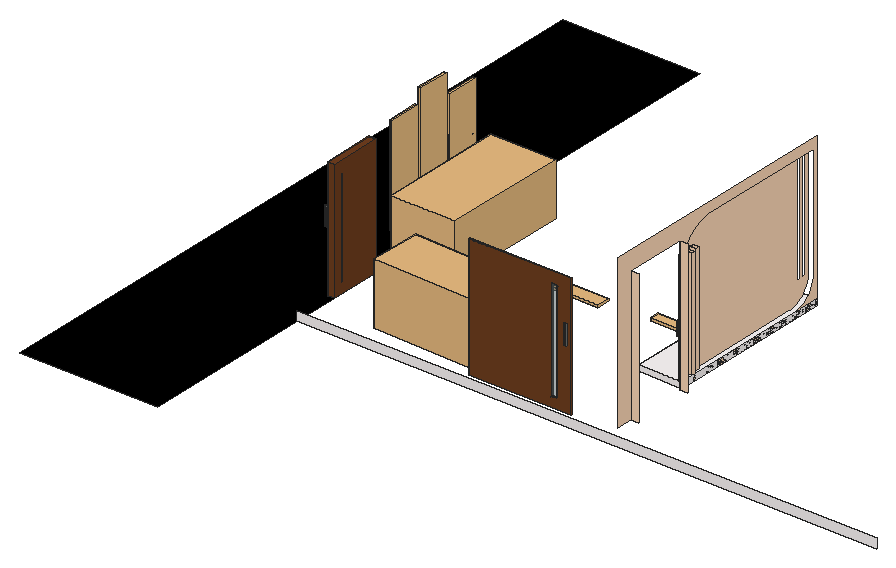
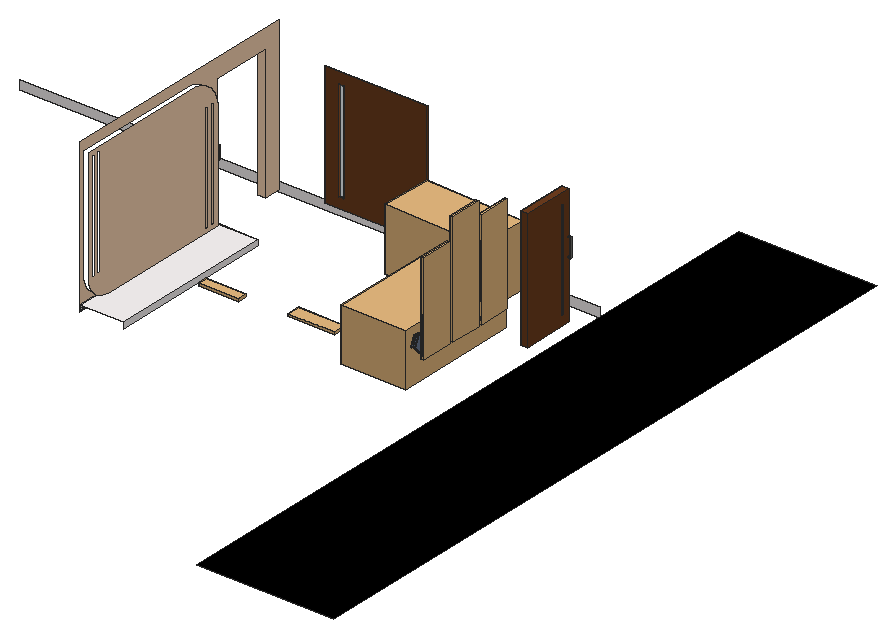
# SketchUp Ruby script. Lengths in inches.
U = 1.inch
M = Sketchup.active_model
def pt(a) = Geom::Point3d.new(a.map { |v| v * U })
def face(e, loops, mat)
  f = e.add_face(loops[0].map { |a| pt(a) })
  loops[1..].each { |l| e.add_face(l.map { |a| pt(a) }).erase! }
  f.material = f.back_material = mat if mat
  f
end
# faces: each face lists its corners as indices into pts; further lists are holes
def faces(e, pts, list, mat = nil) = list.each { |f| face(e, (f[0].is_a?(Array) ? f : [f]).map { |l| l.map { |i| pts[i] } }, mat) }
# xy, xz, yz: faces in a plane at the given z, y or x. An outline is a flat list of corners, or four numbers for a rectangle; further outlines are holes
def ring(l) = l.size == 4 ? [[l[0], l[1]], [l[2], l[1]], [l[2], l[3]], [l[0], l[3]]] : l.each_slice(2).to_a
def flat(e, list, mat, &to3) = list.each { |f| face(e, (f[0].is_a?(Array) ? f : [f]).map { |l| ring(l).map { |u, v| to3.(u, v) } }, mat) }
def xy(e, z, list, mat = nil) = flat(e, list, mat) { |x, y| [x, y, z] }
def xz(e, y, list, mat = nil) = flat(e, list, mat) { |x, z| [x, y, z] }
def yz(e, x, list, mat = nil) = flat(e, list, mat) { |y, z| [x, y, z] }
def lines(e, pts, list) = list.each { |a, b| e.add_line(pt(pts[a]), pt(pts[b])) }
# prism: a flat outline (further loops are holes) pulled along v
def prism(e, loops, v, mat = nil)
  f = face(e, loops, mat); d = Geom::Vector3d.new(v.map { |x| x * U })
  f.pushpull(f.normal.samedirection?(d) ? d.length : -d.length)
end
def box(e, o, s, mat = nil) = prism(e, [[o, [o[0] + s[0], o[1], o[2]], [o[0] + s[0], o[1] + s[1], o[2]], [o[0], o[1] + s[1], o[2]]]], [0, 0, s[2]], mat)
def at(x, y, z, deg = 0) = Geom::Transformation.translation(pt([x, y, z])) * Geom::Transformation.rotation(ORIGIN, Z_AXIS, deg.degrees)
def axes(o, x, y, z) = Geom::Transformation.new([*x, 0, *y, 0, *z, 0, *pt(o).to_a, 1])
def part(name) = M.definitions.add(name)
# library, detail: a bought-in or finely detailed component or shape, given as its bounding box
def library(name, o, s) = part(name).tap { |d| box(d.entities, o, s) }
def detail(e, o, s) = box(e.add_group.entities, o, s)
def put(e, d, t, mat = nil) = e.add_instance(d, t).tap { |i| i.material = mat if mat }
def group(e, t, mat = nil) = e.add_group.tap { |g| g.transformation = t; g.material = mat if mat }.entities
root = M.entities
M.materials.add("3D66_SU_1584934530570_001").color = [198, 166, 120]
M.materials.add("3D66_SU_1584934530605_002").color = [112, 126, 151]
M.materials.add("Material \#1").color = [140, 140, 140]
M.materials.add("[0006_Pink]").color = [255, 192, 203]
M.materials.add("[0010_Snow]").color = [255, 250, 250]
M.materials.add("[0027_PeachPuff]").color = [255, 218, 185]
M.materials.add("[0093_AliceBlue]").color = [240, 248, 255]
M.materials.add("[0137_Black]").color = [0, 0, 0]
M.materials.add("[Metal_Seamed]").color = [118, 119, 115]
M.materials.add("[Translucent_Glass_Safety]").color = [93, 108, 112]
M.materials["[Translucent_Glass_Safety]"].alpha = 0.5
M.materials.add("[Wood_Cherry_Original]").color = [112, 63, 31]
M.materials.add("[Wood_Cherry_Original]1").color = [152, 86, 42]
c1 = part("\#51")
xy(c1.entities,-100.5,[[4942.73,3813.38,5299.1,3883.7]],"3D66_SU_1584934530570_001")
xy(c1.entities,-87.5,[[4944.6875,3815.34,5297.14,3881.74]],"3D66_SU_1584934530570_001")
xz(c1.entities,3813.38,[[4942.73,-100.5,5299.1,-90.5]],"3D66_SU_1584934530570_001")
xz(c1.entities,3883.7,[[4942.73,-100.5,5299.1,-90.5]],"3D66_SU_1584934530570_001")
yz(c1.entities,4942.73,[[3813.38,-100.5,3883.7,-90.5]],"3D66_SU_1584934530570_001")
yz(c1.entities,5299.1,[[3813.38,-100.5,3883.7,-90.5]],"3D66_SU_1584934530570_001")
p = [[4942.73,3883.7,-90.5],[4942.73,3813.38,-90.5],[4944.6875,3815.34,-87.5],[4944.6875,3881.74,-87.5],[5299.1,3813.38,-90.5],[5297.14,3815.34,-87.5],
  [5299.1,3883.7,-90.5],[5297.14,3881.74,-87.5]]
faces(c1.entities,p,[[0,1,2,3],[1,4,5,2],[4,6,7,5],[6,0,3,7]],"3D66_SU_1584934530570_001")
c2 = part("\#48")
xy(c2.entities,-100.5,[[5355.9,3811.42,5712.27,3881.74]],"3D66_SU_1584934530570_001")
xy(c2.entities,-87.5,[[5357.86,3813.38,5710.31,3879.78]],"3D66_SU_1584934530570_001")
xz(c2.entities,3811.42,[[5355.9,-100.5,5712.27,-90.5]],"3D66_SU_1584934530570_001")
xz(c2.entities,3881.74,[[5355.9,-100.5,5712.27,-90.5]],"3D66_SU_1584934530570_001")
yz(c2.entities,5355.9,[[3811.42,-100.5,3881.74,-90.5]],"3D66_SU_1584934530570_001")
yz(c2.entities,5712.27,[[3811.42,-100.5,3881.74,-90.5]],"3D66_SU_1584934530570_001")
p = [[5355.9,3881.74,-90.5],[5355.9,3811.42,-90.5],[5357.86,3813.38,-87.5],[5357.86,3879.78,-87.5],[5712.27,3811.42,-90.5],[5710.31,3813.38,-87.5],
  [5712.27,3881.74,-90.5],[5710.31,3879.78,-87.5]]
faces(c2.entities,p,[[0,1,2,3],[1,4,5,2],[4,6,7,5],[6,0,3,7]],"3D66_SU_1584934530570_001")
c3 = part("\#50")
xy(c3.entities,-100.5,[[4526.8,3811.42,4883.17,3881.74]],"3D66_SU_1584934530570_001")
xy(c3.entities,-87.5,[[4528.76,3813.38,4881.21,3879.78]],"3D66_SU_1584934530570_001")
xz(c3.entities,3811.42,[[4526.8,-100.5,4883.17,-90.5]],"3D66_SU_1584934530570_001")
xz(c3.entities,3881.74,[[4526.8,-100.5,4883.17,-90.5]],"3D66_SU_1584934530570_001")
yz(c3.entities,4526.8,[[3811.42,-100.5,3881.74,-90.5]],"3D66_SU_1584934530570_001")
yz(c3.entities,4883.17,[[3811.42,-100.5,3881.74,-90.5]],"3D66_SU_1584934530570_001")
p = [[4526.8,3881.74,-90.5],[4526.8,3811.42,-90.5],[4528.76,3813.38,-87.5],[4528.76,3879.78,-87.5],[4883.17,3811.42,-90.5],[4881.21,3813.38,-87.5],
  [4883.17,3881.74,-90.5],[4881.21,3879.78,-87.5]]
faces(c3.entities,p,[[0,1,2,3],[1,4,5,2],[4,6,7,5],[6,0,3,7]],"3D66_SU_1584934530570_001")
c4 = library("\#53",[4936.19,3775.67,-115.5],[369.44,1553.17,40])
c5 = part("\#54")
xy(c5.entities,-100.5,[[4523.53,3883.7,4523.53,4334.05,4764.99,3927.74],[4523.53,3883.7,4764.99,3927.74,4784.14,3902.18],[4523.53,3883.7,4784.14,3902.18,4810.21,3883.7],[4810.21,3883.7,4784.14,3902.18,4796.42,3891.95],[4784.14,3902.18,4764.99,3927.74,4773.59,3914.1875],
  [4764.99,3927.74,4523.53,4334.05,4758.58,3942.61],[4758.58,3942.61,4523.53,4334.05,4753.18,3975.46],[4758.58,3942.61,4753.18,3975.46,4754.5625,3958.6],[4753.18,3975.46,4523.53,4334.05,4763.59,4020.47],[4753.18,3975.46,4763.59,4020.47,4755.88,3998.93],
  [4763.59,4020.47,4523.53,4334.05,4791.55,4055.35],[4763.59,4020.47,4791.55,4055.35,4775.6875,4039.49],[4791.55,4055.35,4523.53,4334.05,4810.57,4067.45],[4810.57,4067.45,4523.53,4334.05,4576.49,4391.14],[4810.57,4067.45,4576.49,4391.14,4590.02,4403.74],
  [4810.57,4067.45,4590.02,4403.74,4602.85,4414.71],[4810.57,4067.45,4602.85,4414.71,4615.42,4424.5],[4810.57,4067.45,4615.42,4424.5,4832.11,4075.16],[4886.4375,4072.72,4877.97,4075.17,4886.4375,4525.64],[4886.4375,4072.72,4882.24,4074.03,4877.97,4075.17],
  [4832.11,4075.16,4615.42,4424.5,4621.74,4429.1],[4832.11,4075.16,4621.74,4429.1,4751.37,4455.56],[4832.11,4075.16,4751.37,4455.56,4757.04,4455.48],[4832.11,4075.16,4757.04,4455.48,4855.58,4077.86],[4877.97,4075.17,4869.21,4076.87,4886.4375,4525.64],
  [4877.97,4075.17,4873.62,4076.11,4869.21,4076.87],[4869.21,4076.87,4864.73,4077.42,4878.33,4525.53],[4869.21,4076.87,4878.33,4525.53,4886.4375,4525.64],[4864.73,4077.42,4774.17,4465.69,4785.3,4478.83],[4864.73,4077.42,4860.1875,4077.75,4774.17,4465.69],
  [4864.73,4077.42,4785.3,4478.83,4796.13,4491.95],[4864.73,4077.42,4796.13,4491.95,4806.47,4501.28],[4864.73,4077.42,4806.47,4501.28,4815.83,4508.4],[4864.73,4077.42,4815.83,4508.4,4825.32,4514.1],[4864.73,4077.42,4825.32,4514.1,4836.28,4518.65],
  [4864.73,4077.42,4836.28,4518.65,4849.05,4522.14],[4864.73,4077.42,4849.05,4522.14,4863.07,4524.43],[4864.73,4077.42,4863.07,4524.43,4878.33,4525.53],[4860.1875,4077.75,4768.5,4460.51,4774.17,4465.69],[4860.1875,4077.75,4855.58,4077.86,4768.5,4460.51],
  [4855.58,4077.86,4757.04,4455.48,4762.76,4457],[4855.58,4077.86,4762.76,4457,4768.5,4460.51],[4576.49,4391.14,4583.37,4397.68,4590.02,4403.74],[4590.02,4403.74,4596.5,4409.4,4602.85,4414.71],[4602.85,4414.71,4609.14,4419.72,4615.42,4424.5],
  [4621.74,4429.1,4627.98,4433.56,4751.37,4455.56],[4627.98,4433.56,4634.04,4437.82,4640.03,4441.85],[4627.98,4433.56,4640.03,4441.85,4745.65,4456.74],[4627.98,4433.56,4745.65,4456.74,4751.37,4455.56],[4640.03,4441.85,4646.07,4445.59,4652.26,4449],
  [4640.03,4441.85,4652.26,4449,4745.65,4456.74],[4652.26,4449,4658.73,4452.02,4665.57,4454.62],[4652.26,4449,4665.57,4454.62,4745.65,4456.74],[4665.57,4454.62,4672.96,4456.75,4680.875,4458.47],[4665.57,4454.62,4680.875,4458.47,4745.65,4456.74],
  [4745.65,4456.74,4680.875,4458.47,4697.39,4460.8],[4745.65,4456.74,4697.39,4460.8,4739.8125,4458.5],[4680.875,4458.47,4689.09,4459.8,4697.39,4460.8],[4739.8125,4458.5,4697.39,4460.8,4705.5625,4461.51],[4739.8125,4458.5,4705.5625,4461.51,4733.76,4460.34],
  [4733.76,4460.34,4705.5625,4461.51,4713.4,4461.97],[4733.76,4460.34,4713.4,4461.97,4727.42,4461.75],[4727.42,4461.75,4713.4,4461.97,4720.69,4462.22],[4774.17,4465.69,4779.77,4471.99,4785.3,4478.83],[4785.3,4478.83,4790.76,4485.67,4796.13,4491.95],
  [4796.13,4491.95,4801.43,4497.1,4806.47,4501.28],[4806.47,4501.28,4811.22,4505.04,4815.83,4508.4],[4815.83,4508.4,4820.48,4511.41,4825.32,4514.1],[4825.32,4514.1,4830.54,4516.5,4836.28,4518.65],[4836.28,4518.65,4842.51,4520.54,4849.05,4522.14],
  [4849.05,4522.14,4855.9,4523.43,4863.07,4524.43],[4863.07,4524.43,4870.55,4525.13,4878.33,4525.53]],"3D66_SU_1584934530605_002")
xy(c5.entities,-90.5,[[4523.53,3883.7,4764.99,3927.74,4523.53,4334.05],[4523.53,3883.7,4784.14,3902.18,4764.99,3927.74],[4523.53,3883.7,4810.21,3883.7,4784.14,3902.18],[4810.21,3883.7,4796.42,3891.95,4784.14,3902.18],[4784.14,3902.18,4773.59,3914.1875,4764.99,3927.74],
  [4764.99,3927.74,4758.58,3942.61,4523.53,4334.05],[4758.58,3942.61,4753.18,3975.46,4523.53,4334.05],[4758.58,3942.61,4754.5625,3958.6,4753.18,3975.46],[4753.18,3975.46,4763.59,4020.47,4523.53,4334.05],[4753.18,3975.46,4755.88,3998.93,4763.59,4020.47],
  [4763.59,4020.47,4791.55,4055.35,4523.53,4334.05],[4763.59,4020.47,4775.6875,4039.49,4791.55,4055.35],[4791.55,4055.35,4810.57,4067.45,4523.53,4334.05],[4810.57,4067.45,4576.49,4391.14,4523.53,4334.05],[4810.57,4067.45,4590.02,4403.74,4576.49,4391.14],
  [4810.57,4067.45,4602.85,4414.71,4590.02,4403.74],[4810.57,4067.45,4615.42,4424.5,4602.85,4414.71],[4810.57,4067.45,4832.11,4075.16,4615.42,4424.5],[4886.4375,4072.72,4877.97,4075.17,4882.24,4074.03],[4886.4375,4072.72,4886.4375,4525.64,4877.97,4075.17],
  [4832.11,4075.16,4621.74,4429.1,4615.42,4424.5],[4832.11,4075.16,4751.37,4455.56,4621.74,4429.1],[4832.11,4075.16,4757.04,4455.48,4751.37,4455.56],[4832.11,4075.16,4855.58,4077.86,4757.04,4455.48],[4877.97,4075.17,4869.21,4076.87,4873.62,4076.11],
  [4877.97,4075.17,4886.4375,4525.64,4869.21,4076.87],[4869.21,4076.87,4878.33,4525.53,4864.73,4077.42],[4869.21,4076.87,4886.4375,4525.64,4878.33,4525.53],[4864.73,4077.42,4774.17,4465.69,4860.1875,4077.75],[4864.73,4077.42,4785.3,4478.83,4774.17,4465.69],
  [4864.73,4077.42,4796.13,4491.95,4785.3,4478.83],[4864.73,4077.42,4806.47,4501.28,4796.13,4491.95],[4864.73,4077.42,4815.83,4508.4,4806.47,4501.28],[4864.73,4077.42,4825.32,4514.1,4815.83,4508.4],[4864.73,4077.42,4836.28,4518.65,4825.32,4514.1],
  [4864.73,4077.42,4849.05,4522.14,4836.28,4518.65],[4864.73,4077.42,4863.07,4524.43,4849.05,4522.14],[4864.73,4077.42,4878.33,4525.53,4863.07,4524.43],[4860.1875,4077.75,4768.5,4460.51,4855.58,4077.86],[4860.1875,4077.75,4774.17,4465.69,4768.5,4460.51],
  [4855.58,4077.86,4762.76,4457,4757.04,4455.48],[4855.58,4077.86,4768.5,4460.51,4762.76,4457],[4576.49,4391.14,4590.02,4403.74,4583.37,4397.68],[4590.02,4403.74,4602.85,4414.71,4596.5,4409.4],[4602.85,4414.71,4615.42,4424.5,4609.14,4419.72],
  [4621.74,4429.1,4751.37,4455.56,4627.98,4433.56],[4627.98,4433.56,4640.03,4441.85,4634.04,4437.82],[4627.98,4433.56,4745.65,4456.74,4640.03,4441.85],[4627.98,4433.56,4751.37,4455.56,4745.65,4456.74],[4640.03,4441.85,4652.26,4449,4646.07,4445.59],
  [4640.03,4441.85,4745.65,4456.74,4652.26,4449],[4652.26,4449,4665.57,4454.62,4658.73,4452.02],[4652.26,4449,4745.65,4456.74,4665.57,4454.62],[4665.57,4454.62,4680.875,4458.47,4672.96,4456.75],[4665.57,4454.62,4745.65,4456.74,4680.875,4458.47],
  [4745.65,4456.74,4697.39,4460.8,4680.875,4458.47],[4745.65,4456.74,4739.8125,4458.5,4697.39,4460.8],[4680.875,4458.47,4697.39,4460.8,4689.09,4459.8],[4739.8125,4458.5,4705.5625,4461.51,4697.39,4460.8],[4739.8125,4458.5,4733.76,4460.34,4705.5625,4461.51],
  [4733.76,4460.34,4713.4,4461.97,4705.5625,4461.51],[4733.76,4460.34,4727.42,4461.75,4713.4,4461.97],[4727.42,4461.75,4720.69,4462.22,4713.4,4461.97],[4774.17,4465.69,4785.3,4478.83,4779.77,4471.99],[4785.3,4478.83,4796.13,4491.95,4790.76,4485.67],
  [4796.13,4491.95,4806.47,4501.28,4801.43,4497.1],[4806.47,4501.28,4815.83,4508.4,4811.22,4505.04],[4815.83,4508.4,4825.32,4514.1,4820.48,4511.41],[4825.32,4514.1,4836.28,4518.65,4830.54,4516.5],[4836.28,4518.65,4849.05,4522.14,4842.51,4520.54],
  [4849.05,4522.14,4863.07,4524.43,4855.9,4523.43],[4863.07,4524.43,4878.33,4525.53,4870.55,4525.13]],"3D66_SU_1584934530605_002")
xz(c5.entities,3883.7,[[4523.53,-100.5,4810.21,-100.5,4810.21,-90.5],[4523.53,-100.5,4810.21,-90.5,4523.53,-90.5]],"3D66_SU_1584934530605_002")
yz(c5.entities,4523.53,[[3883.7,-100.5,3883.7,-90.5,4334.05,-100.5],[4334.05,-100.5,3883.7,-90.5,4334.05,-90.5]],"3D66_SU_1584934530605_002")
yz(c5.entities,4886.4375,[[4072.72,-100.5,4525.64,-90.5]],"3D66_SU_1584934530605_002")
p = [[4810.21,3883.7,-90.5],[4810.21,3883.7,-100.5],[4796.42,3891.95,-100.5],[4796.42,3891.95,-90.5],[4784.14,3902.18,-100.5],[4784.14,3902.18,-90.5],
  [4773.59,3914.1875,-100.5],[4773.59,3914.1875,-90.5],[4764.99,3927.74,-100.5],[4764.99,3927.74,-90.5],[4758.58,3942.61,-100.5],[4758.58,3942.61,-90.5],
  [4754.5625,3958.6,-100.5],[4754.5625,3958.6,-90.5],[4753.18,3975.46,-100.5],[4753.18,3975.46,-90.5],[4755.88,3998.93,-100.5],[4755.88,3998.93,-90.5],
  [4763.59,4020.47,-100.5],[4763.59,4020.47,-90.5],[4775.6875,4039.49,-100.5],[4775.6875,4039.49,-90.5],[4791.55,4055.35,-100.5],[4791.55,4055.35,-90.5],
  [4810.57,4067.45,-100.5],[4810.57,4067.45,-90.5],[4832.11,4075.16,-100.5],[4832.11,4075.16,-90.5],[4882.24,4074.03,-90.5],[4882.24,4074.03,-100.5],
  [4886.4375,4072.72,-100.5],[4886.4375,4072.72,-90.5],[4877.97,4075.17,-90.5],[4877.97,4075.17,-100.5],[4855.58,4077.86,-100.5],[4855.58,4077.86,-90.5],
  [4873.62,4076.11,-90.5],[4873.62,4076.11,-100.5],[4869.21,4076.87,-90.5],[4869.21,4076.87,-100.5],[4864.73,4077.42,-90.5],[4864.73,4077.42,-100.5],
  [4860.1875,4077.75,-90.5],[4860.1875,4077.75,-100.5],[4576.49,4391.14,-90.5],[4576.49,4391.14,-100.5],[4523.53,4334.05,-100.5],[4523.53,4334.05,-90.5],
  [4583.37,4397.68,-90.5],[4583.37,4397.68,-100.5],[4590.02,4403.74,-90.5],[4590.02,4403.74,-100.5],[4596.5,4409.4,-90.5],[4596.5,4409.4,-100.5],
  [4602.85,4414.71,-90.5],[4602.85,4414.71,-100.5],[4609.14,4419.72,-90.5],[4609.14,4419.72,-100.5],[4615.42,4424.5,-90.5],[4615.42,4424.5,-100.5],
  [4621.74,4429.1,-90.5],[4621.74,4429.1,-100.5],[4627.98,4433.56,-90.5],[4627.98,4433.56,-100.5],[4634.04,4437.82,-90.5],[4634.04,4437.82,-100.5],
  [4640.03,4441.85,-90.5],[4640.03,4441.85,-100.5],[4646.07,4445.59,-90.5],[4646.07,4445.59,-100.5],[4652.26,4449,-90.5],[4652.26,4449,-100.5],
  [4658.73,4452.02,-90.5],[4658.73,4452.02,-100.5],[4665.57,4454.62,-90.5],[4665.57,4454.62,-100.5],[4672.96,4456.75,-90.5],[4672.96,4456.75,-100.5],
  [4757.04,4455.48,-90.5],[4757.04,4455.48,-100.5],[4751.37,4455.56,-100.5],[4751.37,4455.56,-90.5],[4762.76,4457,-90.5],[4762.76,4457,-100.5],
  [4745.65,4456.74,-100.5],[4745.65,4456.74,-90.5],[4739.8125,4458.5,-100.5],[4739.8125,4458.5,-90.5],[4680.875,4458.47,-90.5],[4680.875,4458.47,-100.5],
  [4768.5,4460.51,-90.5],[4768.5,4460.51,-100.5],[4689.09,4459.8,-90.5],[4689.09,4459.8,-100.5],[4733.76,4460.34,-100.5],[4733.76,4460.34,-90.5],
  [4697.39,4460.8,-90.5],[4697.39,4460.8,-100.5],[4727.42,4461.75,-100.5],[4727.42,4461.75,-90.5],[4774.17,4465.69,-90.5],[4774.17,4465.69,-100.5],
  [4705.5625,4461.51,-90.5],[4705.5625,4461.51,-100.5],[4713.4,4461.97,-90.5],[4713.4,4461.97,-100.5],[4720.69,4462.22,-100.5],[4720.69,4462.22,-90.5],
  [4779.77,4471.99,-90.5],[4779.77,4471.99,-100.5],[4785.3,4478.83,-90.5],[4785.3,4478.83,-100.5],[4790.76,4485.67,-90.5],[4790.76,4485.67,-100.5],
  [4796.13,4491.95,-90.5],[4796.13,4491.95,-100.5],[4801.43,4497.1,-90.5],[4801.43,4497.1,-100.5],[4806.47,4501.28,-90.5],[4806.47,4501.28,-100.5],
  [4811.22,4505.04,-90.5],[4811.22,4505.04,-100.5],[4815.83,4508.4,-90.5],[4815.83,4508.4,-100.5],[4820.48,4511.41,-90.5],[4820.48,4511.41,-100.5],
  [4825.32,4514.1,-90.5],[4825.32,4514.1,-100.5],[4830.54,4516.5,-90.5],[4830.54,4516.5,-100.5],[4836.28,4518.65,-90.5],[4836.28,4518.65,-100.5],
  [4842.51,4520.54,-90.5],[4842.51,4520.54,-100.5],[4849.05,4522.14,-90.5],[4849.05,4522.14,-100.5],[4855.9,4523.43,-90.5],[4855.9,4523.43,-100.5],
  [4863.07,4524.43,-90.5],[4863.07,4524.43,-100.5],[4870.55,4525.13,-90.5],[4870.55,4525.13,-100.5],[4878.33,4525.53,-90.5],[4878.33,4525.53,-100.5],
  [4886.4375,4525.64,-90.5],[4886.4375,4525.64,-100.5]]
faces(c5.entities,p,[[0,1,2,3],[3,2,4,5],[5,4,6,7],[7,6,8,9],[9,8,10,11],[11,10,12,13],[13,12,14,15],[15,14,16,17],
  [17,16,18,19],[19,18,20,21],[21,20,22,23],[23,22,24,25],[25,24,26,27],[28,29,30,31],[32,33,29,28],[27,26,34,35],
  [36,37,33,32],[38,39,37,36],[40,41,39,38],[42,43,41,40],[35,34,43,42],[44,45,46,47],[48,49,45,44],[50,51,49,48],
  [52,53,51,50],[54,55,53,52],[56,57,55,54],[58,59,57,56],[60,61,59,58],[62,63,61,60],[64,65,63,62],[66,67,65,64],
  [68,69,67,66],[70,71,69,68],[72,73,71,70],[74,75,73,72],[76,77,75,74],[78,79,80,81],[82,83,79,78],[81,80,84,85],
  [85,84,86,87],[88,89,77,76],[90,91,83,82],[92,93,89,88],[87,86,94,95],[96,97,93,92],[95,94,98,99],[100,101,91,90],
  [102,103,97,96],[104,105,103,102],[99,98,106,107],[107,106,105,104],[108,109,101,100],[110,111,109,108],[112,113,111,110],[114,115,113,112],
  [116,117,115,114],[118,119,117,116],[120,121,119,118],[122,123,121,120],[124,125,123,122],[126,127,125,124],[128,129,127,126],[130,131,129,128],
  [132,133,131,130],[134,135,133,132],[136,137,135,134],[138,139,137,136],[140,141,139,138],[142,143,141,140],[144,145,143,142]],"3D66_SU_1584934530605_002")
c6 = library("\#47",[5349.36,3775.67,-115.5],[369.44,1364.36,40])
c7 = library("\#46",[4520.26,3775.67,-115.5],[369.44,1264.84,40])
c8 = library("The OG Sofa with Chaise",[-47.49,-31.48,0.03],[94.92,63.03,31.23])
c9 = library("Reva LHF-RHF Double Sofa With Chaise",[-18.375,-7.52,0.07],[74.16,40.55,32.92])
c10 = part("Untitled (1)")
xy(c10.entities,0,[[-637.99,-155.05,-557,-154.04],[-770.21,-130.91,-764.41,-89.48]],"[Wood_Cherry_Original]")
xy(c10.entities,7.92,[[-770.21,-125.17,-767.82,-123.17],[-767.82,-125.17,-764.41,-123.17]],"[Wood_Cherry_Original]")
xy(c10.entities,8.11,[[-572.14,-155.05,-568.23,-154.63],[-572.14,-154.63,-568.23,-154.04]],"[Wood_Cherry_Original]")
xy(c10.entities,47.5,[[-773.63,-129.375,-770.21,-128.48]],"[Wood_Cherry_Original]")
xy(c10.entities,48.47,[[-772.26,-129.375,-770.21,-128.48]],"[Metal_Seamed]")
xy(c10.entities,48.62,[[-561.76,-155.64,-560.01,-155.05]],"[Wood_Cherry_Original]")
xy(c10.entities,49.61,[[-561.76,-155.41,-560.01,-155.05]],"[Metal_Seamed]")
xy(c10.entities,62,[[-772.26,-129.375,-770.21,-128.48]],"[Metal_Seamed]")
xy(c10.entities,62.69,[[-773.63,-129.375,-770.21,-128.48]],"[Wood_Cherry_Original]")
xy(c10.entities,63.46,[[-561.76,-155.41,-560.01,-155.05]],"[Metal_Seamed]")
xy(c10.entities,64.17,[[-561.76,-155.64,-560.01,-155.05]],"[Wood_Cherry_Original]")
xy(c10.entities,86.78,[[-770.21,-125.17,-767.82,-123.17],[-767.82,-125.17,-764.41,-123.17]],"[Wood_Cherry_Original]")
xy(c10.entities,88.82,[[-572.14,-155.05,-568.23,-154.63],[-572.14,-154.63,-568.23,-154.04]],"[Wood_Cherry_Original]")
xy(c10.entities,95.4375,[[-770.21,-130.91,-764.41,-89.48]],"[Wood_Cherry_Original]")
xy(c10.entities,97.6875,[[-637.99,-155.05,-557,-154.04]],"[Wood_Cherry_Original]")
xz(c10.entities,-155.64,[[-561.76,48.62,-560.01,64.17]],"[Metal_Seamed]")
xz(c10.entities,-155.41,[[-561.76,49.61,-560.01,63.46]],"[Metal_Seamed]")
xz(c10.entities,-155.05,[[[-637.99,0,-557,97.6875],[-572.88,7.59,-567.5,89.34],[-561.76,48.62,-560.01,49.61],[-561.76,63.46,-560.01,64.17]],[-572.88,7.59,-567.5,7.59,-567.5,89.34,-572.14,89.34,-572.14,88.82,-568.23,88.82,-568.23,8.11,-572.88,8.11],[-572.88,8.11,-572.14,89.34]],"[Wood_Cherry_Original]")
xz(c10.entities,-154.63,[[-572.14,8.11,-568.23,88.82]],"[Translucent_Glass_Safety]")
xz(c10.entities,-154.04,[[[-637.99,0,-557,97.6875],[-572.14,8.11,-568.23,88.82]]],"[Wood_Cherry_Original]")
xz(c10.entities,-130.91,[[-770.21,0,-764.41,95.4375]],"[Wood_Cherry_Original]")
xz(c10.entities,-129.375,[[-773.63,47.5,-770.21,47.5,-770.21,48.47,-772.26,48.47,-772.26,62,-770.21,62,-770.21,62.69,-773.63,62.69]],"[Metal_Seamed]")
xz(c10.entities,-128.48,[[-773.63,47.5,-773.63,62.69,-770.21,62.69,-770.21,62,-772.26,62,-772.26,48.47,-770.21,48.47,-770.21,47.5]],"[Metal_Seamed]")
xz(c10.entities,-125.17,[[-770.21,7.92,-767.82,86.78]],"[Wood_Cherry_Original]")
xz(c10.entities,-125.17,[[-767.82,7.92,-764.41,86.78]],"[Wood_Cherry_Original]1")
xz(c10.entities,-123.17,[[-770.21,7.92,-767.82,86.78],[-767.82,7.92,-764.41,86.78]],"[Wood_Cherry_Original]")
xz(c10.entities,-89.48,[[-770.21,0,-764.41,95.4375]],"[Wood_Cherry_Original]")
yz(c10.entities,-773.63,[[-129.375,47.5,-128.48,62.69]],"[Metal_Seamed]")
yz(c10.entities,-772.26,[[-129.375,48.47,-128.48,62]],"[Metal_Seamed]")
yz(c10.entities,-770.21,[[[-130.91,0,-89.48,95.4375],[-125.55,7.41,-122.79,87.28],[-129.375,47.5,-128.48,48.47],[-129.375,62,-128.48,62.69]],[-125.55,7.41,-125.55,87.28,-123.17,87.28,-123.17,86.78,-125.17,86.78,-125.17,7.92,-122.79,7.92,-122.79,7.41],[-123.17,7.92,-122.79,87.28]],"[Wood_Cherry_Original]")
yz(c10.entities,-767.82,[[-125.17,7.92,-123.17,86.78]],"[Translucent_Glass_Safety]")
yz(c10.entities,-764.41,[[[-130.91,0,-89.48,95.4375],[-125.17,7.92,-123.17,86.78]]],"[Wood_Cherry_Original]")
yz(c10.entities,-637.99,[[-155.05,0,-154.04,97.6875]],"[Wood_Cherry_Original]")
yz(c10.entities,-572.14,[[-155.05,8.11,-154.63,88.82],[-154.63,8.11,-154.04,88.82]],"[Wood_Cherry_Original]")
yz(c10.entities,-568.23,[[-155.05,8.11,-154.63,88.82]],"[Wood_Cherry_Original]")
yz(c10.entities,-568.23,[[-154.63,8.11,-154.04,88.82]],"[Wood_Cherry_Original]1")
yz(c10.entities,-561.76,[[-155.64,48.62,-155.64,64.17,-155.05,64.17,-155.05,63.46,-155.41,63.46,-155.41,49.61,-155.05,49.61,-155.05,48.62]],"[Metal_Seamed]")
yz(c10.entities,-560.01,[[-155.64,48.62,-155.05,48.62,-155.05,49.61,-155.41,49.61,-155.41,63.46,-155.05,63.46,-155.05,64.17,-155.64,64.17]],"[Metal_Seamed]")
yz(c10.entities,-557,[[-155.05,0,-154.04,97.6875]],"[Wood_Cherry_Original]")
c11 = library("Living ar",[0.98,0,0],[37.37,10.22,2])
c12 = library("TV unit",[0.32,0,0],[31.91,7.8,2])
xy(root,-7.5625,[[0,0.375,109.5625,540.9375]],"[0137_Black]")
xy(root,4.8125,[[323.75,211.625,358.5625,345.9375]],"[0010_Snow]")
xy(root,4.8125,[[354.3125,213.375,358.5625,322.76]],"[0027_PeachPuff]")
xy(root,7.66,[[354.3125,217.7,361.25,220.7],[354.3125,223.77,359.875,226.77]],"[0027_PeachPuff]")
xz(root,138.9375,[[109.5625,-7.5625,571.5625,0]],"[0010_Snow]")
xz(root,160.62,[[358.5625,0,364.5625,106.4375]],"[0027_PeachPuff]")
xz(root,209.49,[[358.5625,0,364.5625,106.4375]],"[0027_PeachPuff]")
xz(root,211.625,[[323.75,0,358.5625,4.8125]],"[0010_Snow]")
xz(root,213.375,[[354.3125,4.8125,358.5625,88.23]],"[0027_PeachPuff]")
xz(root,217.7,[[354.3125,7.66,361.25,94.84]],"[0027_PeachPuff]")
xz(root,220.7,[[354.3125,7.66,361.25,94.84]],"[0027_PeachPuff]")
xz(root,223.77,[[354.3125,7.66,359.875,94.84]],"[0027_PeachPuff]")
xz(root,226.77,[[354.3125,7.66,359.875,94.84]],"[0027_PeachPuff]")
xz(root,241.42,[[122.5,44.6,122.5,88.07,123.07,88.07],[122.5,44.6,123.07,88.07,123.07,44.6]],"3D66_SU_1584934530605_002")
xz(root,302.48,[[122.5,34.47,123.07,48.84]],"3D66_SU_1584934530605_002")
yz(root,122.5,[[302.48,34.47,302.48,48.84,306.56,39.18],[306.56,39.18,302.48,48.84,307.31,39.95],[307.31,39.95,302.48,48.84,307.63,40.27],[307.63,40.27,302.48,48.84,303,48.85],[307.63,40.27,303,48.85,303.52,48.84],
  [307.63,40.27,303.52,48.84,307.93,40.55],[307.93,40.55,303.52,48.84,304.58,48.81],[307.93,40.55,304.58,48.81,308.09,40.68],[308.09,40.68,304.58,48.81,308.24,40.8],[308.24,40.8,304.58,48.81,305.1,48.82],
  [308.24,40.8,305.1,48.82,308.4,40.91],[308.4,40.91,305.1,48.82,308.57,41.02],[308.57,41.02,305.1,48.82,305.36,48.83],[308.57,41.02,305.36,48.83,308.75,41.12],[308.75,41.12,305.36,48.83,305.61,48.85],
  [308.75,41.12,305.61,48.85,308.9375,41.21],[308.9375,41.21,305.61,48.85,305.85,48.88],[308.9375,41.21,305.85,48.88,309.14,41.3],[309.14,41.3,305.85,48.88,306.09,48.92],[309.14,41.3,306.09,48.92,309.36,41.39],
  [309.36,41.39,306.09,48.92,306.33,48.97],[309.59,41.47,306.33,48.97,306.44,49],[309.59,41.47,306.44,49,306.56,49.03],[309.84,41.54,306.56,49.03,306.67,49.07],[310.1,41.6,306.67,49.07,306.78,49.12],
  [310.1,41.6,306.78,49.12,306.88,49.16],[310.375,41.64,306.88,49.16,306.99,49.22],[241.42,44.6,235.3125,49.2,237.76,84.43],[241.42,44.6,237.76,84.43,238.26,84.84],[241.42,44.6,238.26,84.84,239.29,85.85],
  [241.42,44.6,239.29,85.85,240.36,86.97],[241.42,44.6,240.36,86.97,241.42,88.07]],"3D66_SU_1584934530605_002")
yz(root,123.07,[[302.48,34.47,306.56,39.18,302.48,48.84],[306.56,39.18,307.31,39.95,302.48,48.84],[307.31,39.95,307.63,40.27,302.48,48.84],[307.63,40.27,303,48.85,302.48,48.84],[307.63,40.27,303.52,48.84,303,48.85],
  [307.63,40.27,307.93,40.55,303.52,48.84],[307.93,40.55,304.58,48.81,303.52,48.84],[307.93,40.55,308.09,40.68,304.58,48.81],[308.09,40.68,308.24,40.8,304.58,48.81],[308.24,40.8,305.1,48.82,304.58,48.81],
  [308.24,40.8,308.4,40.91,305.1,48.82],[308.4,40.91,308.57,41.02,305.1,48.82],[308.57,41.02,305.36,48.83,305.1,48.82],[308.57,41.02,308.75,41.12,305.36,48.83],[308.75,41.12,305.61,48.85,305.36,48.83],
  [308.75,41.12,308.9375,41.21,305.61,48.85],[308.9375,41.21,305.85,48.88,305.61,48.85],[308.9375,41.21,309.14,41.3,305.85,48.88],[309.14,41.3,306.09,48.92,305.85,48.88],[309.14,41.3,309.36,41.39,306.09,48.92],
  [309.36,41.39,306.33,48.97,306.09,48.92],[309.59,41.47,306.44,49,306.33,48.97],[309.59,41.47,306.56,49.03,306.44,49],[309.84,41.54,306.67,49.07,306.56,49.03],[310.1,41.6,306.78,49.12,306.67,49.07],
  [310.1,41.6,306.88,49.16,306.78,49.12],[310.375,41.64,306.99,49.22,306.88,49.16],[241.42,44.6,237.76,84.43,235.3125,49.2],[241.42,44.6,238.26,84.84,237.76,84.43],[241.42,44.6,239.29,85.85,238.26,84.84],
  [241.42,44.6,240.36,86.97,239.29,85.85],[241.42,44.6,241.42,88.07,240.36,86.97]],"3D66_SU_1584934530605_002")
yz(root,323.75,[[211.625,0,345.9375,4.8125]],"[0010_Snow]")
yz(root,354.3125,[[[213.375,4.8125,213.375,88.23,213.59,91.51,214.23,94.73,215.29,97.85,216.74,100.79,218.57,103.52,220.73,106,223.2,108.16,225.93,109.99,228.88,111.44,231.99,112.5,235.22,113.14,238.49,113.35,342.58,113.35,342.58,24.64,342.42,22.05,341.91,19.51,341.08,17.05,339.93,14.73,338.49,12.57,336.78,10.62,334.83,8.91,332.67,7.47,330.34,6.32,327.89,5.49,325.34,4.98,322.76,4.8125],[336.47,23.08,339.47,110.27],[330.97,23.08,333.97,110.27],[217.7,7.66,220.7,94.84],[223.77,7.66,226.77,94.84]]],"[0027_PeachPuff]")
yz(root,358.5625,[[211.625,0,345.9375,4.8125]],"[0010_Snow]")
yz(root,358.5625,[[[147.9375,0,147.9375,121.1875,345.9375,121.1875,345.9375,0,209.49,0,209.49,106.4375,160.62,106.4375,160.62,0],[213.375,4.8125,322.76,4.8125,325.34,4.98,327.89,5.49,330.34,6.32,332.67,7.47,334.83,8.91,336.78,10.62,338.49,12.57,339.93,14.73,341.08,17.05,341.91,19.51,342.42,22.05,342.58,24.64,342.58,113.35,238.49,113.35,235.22,113.14,231.99,112.5,228.88,111.44,225.93,109.99,223.2,108.16,220.73,106,218.57,103.52,216.74,100.79,215.29,97.85,214.23,94.73,213.59,91.51,213.375,88.23]]],"[0027_PeachPuff]")
yz(root,359.875,[[223.77,7.66,226.77,94.84]],"[0027_PeachPuff]")
yz(root,361.25,[[217.7,7.66,220.7,94.84]],"[0027_PeachPuff]")
yz(root,362.57,[[201.8,43.52,201.66,43.55,201.66,43.53],[201.8,43.52,201.8,43.53,201.66,43.55],[201.8,43.52,201.94,43.53,201.8,43.53],[201.66,43.53,201.53,43.59,201.52,43.57],[201.66,43.53,201.66,43.55,201.53,43.59],
  [201.8,43.53,201.94,43.53,201.9375,43.55],[201.9375,43.55,202.07,43.57,202.07,43.59],[201.52,43.57,201.41,43.65,201.4,43.64],[201.52,43.57,201.53,43.59,201.41,43.65],[202.07,43.57,202.2,43.64,202.07,43.59],
  [202.07,43.59,202.2,43.64,202.19,43.65],[201.4,43.64,201.3,43.73,201.29,43.72],[201.4,43.64,201.41,43.65,201.3,43.73],[202.2,43.64,202.31,43.72,202.19,43.65],[202.19,43.65,202.31,43.72,202.3,43.73],
  [201.29,43.72,201.2,43.83,201.19,43.83],[201.29,43.72,201.3,43.73,201.2,43.83],[202.31,43.72,202.4,43.83,202.3,43.73],[202.3,43.73,202.4,43.83,202.39,43.83],[201.75,43.75,201.71,43.78,201.71,43.77],
  [201.75,43.75,201.75,43.77,201.71,43.78],[201.75,43.75,201.8,43.75,201.75,43.77],[201.8,43.75,201.8,43.76,201.75,43.77],[201.8,43.75,201.84,43.75,201.8,43.76],[201.84,43.75,201.84,43.77,201.8,43.76],
  [201.84,43.75,201.89,43.77,201.84,43.77],[201.71,43.77,201.67,43.8,201.67,43.79],[201.71,43.77,201.71,43.78,201.67,43.8],[201.84,43.77,201.89,43.77,201.88,43.78],[201.89,43.77,201.93,43.79,201.88,43.78],
  [201.88,43.78,201.93,43.79,201.92,43.8],[201.67,43.79,201.64,43.83,201.63,43.82],[201.67,43.79,201.67,43.8,201.64,43.83],[201.63,43.82,201.61,43.86,201.6,43.85],[201.63,43.82,201.64,43.83,201.61,43.86],
  [201.19,43.83,201.2,43.83,201.125,43.95],[201.6,43.85,201.58,43.9,201.57,43.89],[201.6,43.85,201.61,43.86,201.58,43.9],[201.57,43.89,201.5625,43.94,201.55,43.9375],[201.57,43.89,201.58,43.9,201.5625,43.94],
  [201.55,43.9375,201.55,43.99,201.54,43.98],[201.55,43.9375,201.5625,43.94,201.55,43.99],[202.47,43.95,202.54,44.08,202.53,44.09],[201.54,43.98,201.55,44.04,201.53,44.04],[201.54,43.98,201.55,43.99,201.55,44.04],
  [201.53,44.04,201.55,44.04,201.55,44.08],[201.53,44.04,201.55,44.08,201.54,44.09],[201.06,44.08,201.03,44.23,201.02,44.23],[201.55,44.08,201.5625,44.13,201.54,44.09],[202.54,44.08,202.58,44.23,202.53,44.09],
  [201.54,44.09,201.5625,44.13,201.55,44.14],[202.53,44.09,202.58,44.23,202.5625,44.23],[201.5625,44.13,201.58,44.17,201.55,44.14],[201.55,44.14,201.58,44.17,201.57,44.18],[201.58,44.17,201.61,44.21,201.57,44.18],
  [201.57,44.18,201.61,44.21,201.6,44.22],[201.61,44.21,201.64,44.24,201.6,44.22],[201.6,44.22,201.64,44.24,201.63,44.25],[201.02,44.23,201.02,44.39,201.01,44.39],[201.02,44.23,201.03,44.23,201.02,44.39],
  [202.5625,44.23,202.58,44.23,202.59,44.39],[202.5625,44.23,202.59,44.39,202.58,44.39],[201.64,44.24,201.67,44.27,201.63,44.25],[201.63,44.25,201.67,44.27,201.67,44.28],[201.67,44.27,201.71,44.29,201.67,44.28],
  [201.92,44.27,201.89,44.3,201.88,44.29],[201.67,44.28,201.71,44.29,201.71,44.3],[201.71,44.29,201.75,44.3,201.71,44.3],[201.88,44.29,201.84,44.32,201.84,44.3],[201.88,44.29,201.89,44.3,201.84,44.32],
  [201.71,44.3,201.75,44.3,201.75,44.32],[201.75,44.3,201.8,44.31,201.75,44.32],[201.84,44.3,201.8,44.32,201.8,44.31],[201.84,44.3,201.84,44.32,201.8,44.32],[201.8,44.31,201.8,44.32,201.75,44.32],
  [201.01,44.39,201.02,44.39,201.02,52.11],[201.01,44.39,201.02,52.11,201.02,54.24],[201.01,44.39,201.02,54.24,201.01,54.24],[202.58,44.39,202.59,44.39,202.59,54.24],[202.58,44.39,202.59,54.24,202.58,54.24]],"Material \#1")
p = [[123.07,302.48,34.47],[122.5,302.48,34.47],[122.5,306.56,39.18],[123.07,306.56,39.18],[122.5,307.31,39.95],[123.07,307.31,39.95],
  [122.5,307.63,40.27],[123.07,307.63,40.27],[122.5,307.93,40.55],[123.07,307.93,40.55],[122.5,308.09,40.68],[123.07,308.09,40.68],
  [122.5,308.24,40.8],[123.07,308.24,40.8],[122.5,308.4,40.91],[123.07,308.4,40.91],[122.5,241.42,44.6],[123.07,241.42,44.6],
  [123.07,235.3125,49.2],[122.5,235.3125,49.2]]
faces(root,p,[[0,1,2,3],[3,2,4,5],[5,4,6,7],[7,6,8,9],[9,8,10,11],[11,10,12,13],[13,12,14,15],[16,17,18,19]],"3D66_SU_1584934530605_002")
put(root,c1,axes([117.28,611.37,-189.42],[0,-0.06912,0],[0,0,0.0576],[-0.0576,0,0]),"3D66_SU_1584934530570_001")
put(root,c2,axes([117.28,611.37,-189.42],[0,-0.06912,0],[0,0,0.0576],[-0.0576,0,0]),"3D66_SU_1584934530570_001")
put(root,c3,axes([117.28,611.37,-189.42],[0,-0.06912,0],[0,0,0.0576],[-0.0576,0,0]),"3D66_SU_1584934530570_001")
put(root,c4,axes([117.28,611.37,-189.42],[0,-0.06912,0],[0,0,0.0576],[-0.0576,0,0]),"3D66_SU_1584934530570_001")
put(root,c5,axes([117.28,611.37,-189.42],[0,-0.06912,0],[0,0,0.0576],[-0.0576,0,0]),"3D66_SU_1584934530605_002")
put(root,c6,axes([117.28,611.37,-189.42],[0,-0.06912,0],[0,0,0.0576],[-0.0576,0,0]),"3D66_SU_1584934530570_001")
put(root,c7,axes([117.28,611.37,-189.42],[0,-0.06912,0],[0,0,0.0576],[-0.0576,0,0]),"3D66_SU_1584934530570_001")
put(root,c8,axes([150.17,263.82,12.39],[0,1.053,0],[-0.82,0,0],[0,0,1.35]),"[0093_AliceBlue]")
put(root,c9,axes([220.88,182.73,-0.11],[-1.06572,0.03815,0],[-0.03577,-0.99936,0],[0,0,1.5]),"[0093_AliceBlue]")
put(root,c10,at(882.56,296.85,0),"[0006_Pink]")
put(root,c11,at(215.31,259.24,0))
put(root,c12,at(289.16,266.36,0))
